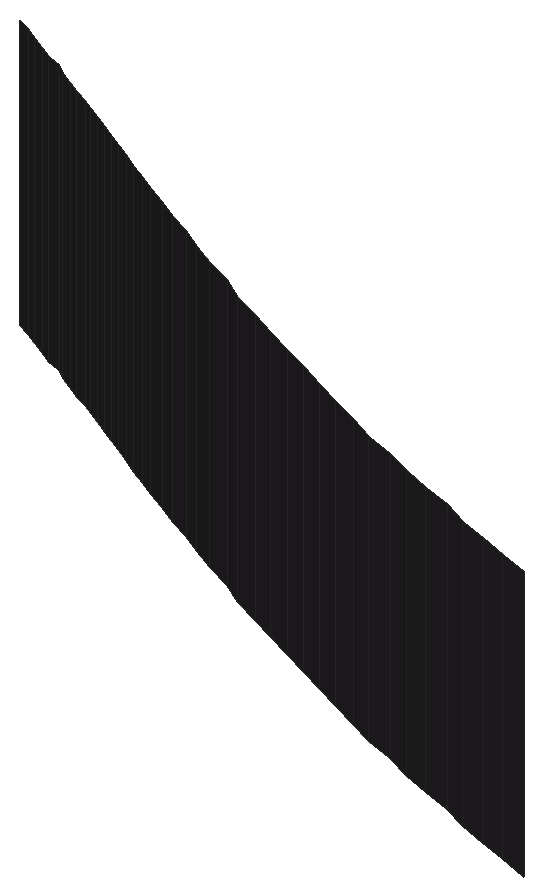
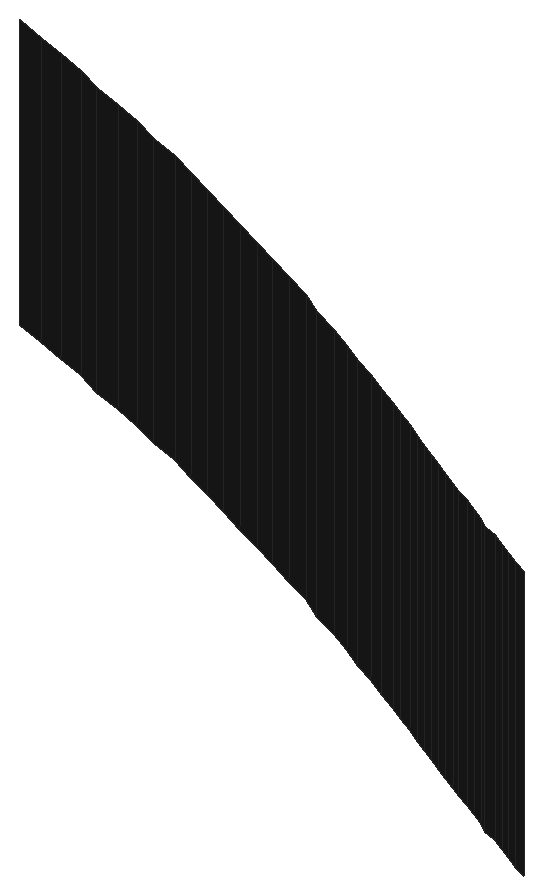
# SketchUp Ruby script. Lengths in inches.
U = 1.inch
M = Sketchup.active_model
def pt(a) = Geom::Point3d.new(a.map { |v| v * U })
def face(e, loops, mat)
  f = e.add_face(loops[0].map { |a| pt(a) })
  loops[1..].each { |l| e.add_face(l.map { |a| pt(a) }).erase! }
  f.material = f.back_material = mat if mat
  f
end
# faces: each face lists its corners as indices into pts; further lists are holes
def faces(e, pts, list, mat = nil) = list.each { |f| face(e, (f[0].is_a?(Array) ? f : [f]).map { |l| l.map { |i| pts[i] } }, mat) }
# xy, xz, yz: faces in a plane at the given z, y or x. An outline is a flat list of corners, or four numbers for a rectangle; further outlines are holes
def ring(l) = l.size == 4 ? [[l[0], l[1]], [l[2], l[1]], [l[2], l[3]], [l[0], l[3]]] : l.each_slice(2).to_a
def flat(e, list, mat, &to3) = list.each { |f| face(e, (f[0].is_a?(Array) ? f : [f]).map { |l| ring(l).map { |u, v| to3.(u, v) } }, mat) }
def xy(e, z, list, mat = nil) = flat(e, list, mat) { |x, y| [x, y, z] }
def xz(e, y, list, mat = nil) = flat(e, list, mat) { |x, z| [x, y, z] }
def yz(e, x, list, mat = nil) = flat(e, list, mat) { |y, z| [x, y, z] }
def lines(e, pts, list) = list.each { |a, b| e.add_line(pt(pts[a]), pt(pts[b])) }
# prism: a flat outline (further loops are holes) pulled along v
def prism(e, loops, v, mat = nil)
  f = face(e, loops, mat); d = Geom::Vector3d.new(v.map { |x| x * U })
  f.pushpull(f.normal.samedirection?(d) ? d.length : -d.length)
end
def box(e, o, s, mat = nil) = prism(e, [[o, [o[0] + s[0], o[1], o[2]], [o[0] + s[0], o[1] + s[1], o[2]], [o[0], o[1] + s[1], o[2]]]], [0, 0, s[2]], mat)
def at(x, y, z, deg = 0) = Geom::Transformation.translation(pt([x, y, z])) * Geom::Transformation.rotation(ORIGIN, Z_AXIS, deg.degrees)
def axes(o, x, y, z) = Geom::Transformation.new([*x, 0, *y, 0, *z, 0, *pt(o).to_a, 1])
def part(name) = M.definitions.add(name)
# library, detail: a bought-in or finely detailed component or shape, given as its bounding box
def library(name, o, s) = part(name).tap { |d| box(d.entities, o, s) }
def detail(e, o, s) = box(e.add_group.entities, o, s)
def put(e, d, t, mat = nil) = e.add_instance(d, t).tap { |i| i.material = mat if mat }
def group(e, t, mat = nil) = e.add_group.tap { |g| g.transformation = t; g.material = mat if mat }.entities
root = M.entities
M.materials.add("Marble_07_1K").color = [36, 34, 36]
p = [[343.27,773.38,18],[343.375,773.34,18],[343.375,773.34,19],[343.27,773.38,19],[343.48,773.3,18],[343.48,773.3,19],
  [343.59,773.26,18],[343.59,773.26,19],[343.0625,773.47,18],[343.17,773.43,18],[343.17,773.43,19],[343.0625,773.47,19],
  [342.86,773.56,18],[342.96,773.51,18],[342.96,773.51,19],[342.86,773.56,19],[342.65,773.65,18],[342.75,773.6,18],
  [342.75,773.6,19],[342.65,773.65,19],[342.35,773.8,18],[342.45,773.75,18],[342.45,773.75,19],[342.35,773.8,19],
  [342.55,773.7,18],[342.55,773.7,19],[342.15,773.9,18],[342.25,773.85,18],[342.25,773.85,19],[342.15,773.9,19],
  [342.05,773.95,18],[342.05,773.95,19],[341.86,774.06,18],[341.95,774,18],[341.95,774,19],[341.86,774.06,19],
  [341.67,774.16,18],[341.76,774.11,18],[341.76,774.11,19],[341.67,774.16,19],[341.51,774.25,18],[341.59,774.21,18],
  [341.59,774.21,19],[341.51,774.25,19],[341.3,774.375,18],[341.36,774.34,18],[341.36,774.34,19],[341.3,774.375,19],
  [341.43,774.3,18],[341.43,774.3,19],[341.13,774.48,18],[341.18,774.45,18],[341.18,774.45,19],[341.13,774.48,19],
  [341.24,774.41,18],[341.24,774.41,19],[340.98,774.57,18],[341.03,774.54,18],[341.03,774.54,19],[340.98,774.57,19],
  [341.08,774.51,18],[341.08,774.51,19],[340.84,774.65,18],[340.89,774.625,18],[340.89,774.625,19],[340.84,774.65,19],
  [340.93,774.6,18],[340.93,774.6,19],[340.65,774.76,18],[340.7,774.74,18],[340.7,774.74,19],[340.65,774.76,19],
  [340.74,774.71,18],[340.74,774.71,19],[340.79,774.68,18],[340.79,774.68,19],[340.45,774.875,18],[340.5,774.85,18],
  [340.5,774.85,19],[340.45,774.875,19],[340.55,774.82,18],[340.55,774.82,19],[340.6,774.79,18],[340.6,774.79,19]]
faces(root,p,[[0,1,2,3],[1,4,5,2],[4,6,7,5],[8,9,10,11],[9,0,3,10],[12,13,14,15],[13,8,11,14],[16,17,18,19],
  [17,12,15,18],[20,21,22,23],[21,24,25,22],[24,16,19,25],[26,27,28,29],[27,20,23,28],[30,26,29,31],[32,33,34,35],
  [33,30,31,34],[36,37,38,39],[37,32,35,38],[40,41,42,43],[41,36,39,42],[44,45,46,47],[45,48,49,46],[48,40,43,49],
  [50,51,52,53],[51,54,55,52],[54,44,47,55],[56,57,58,59],[57,60,61,58],[60,50,53,61],[62,63,64,65],[63,66,67,64],
  [66,56,59,67],[68,69,70,71],[69,72,73,70],[72,74,75,73],[74,62,65,75],[76,77,78,79],[77,80,81,78],[80,82,83,81],
  [82,68,71,83]],"Marble_07_1K")
